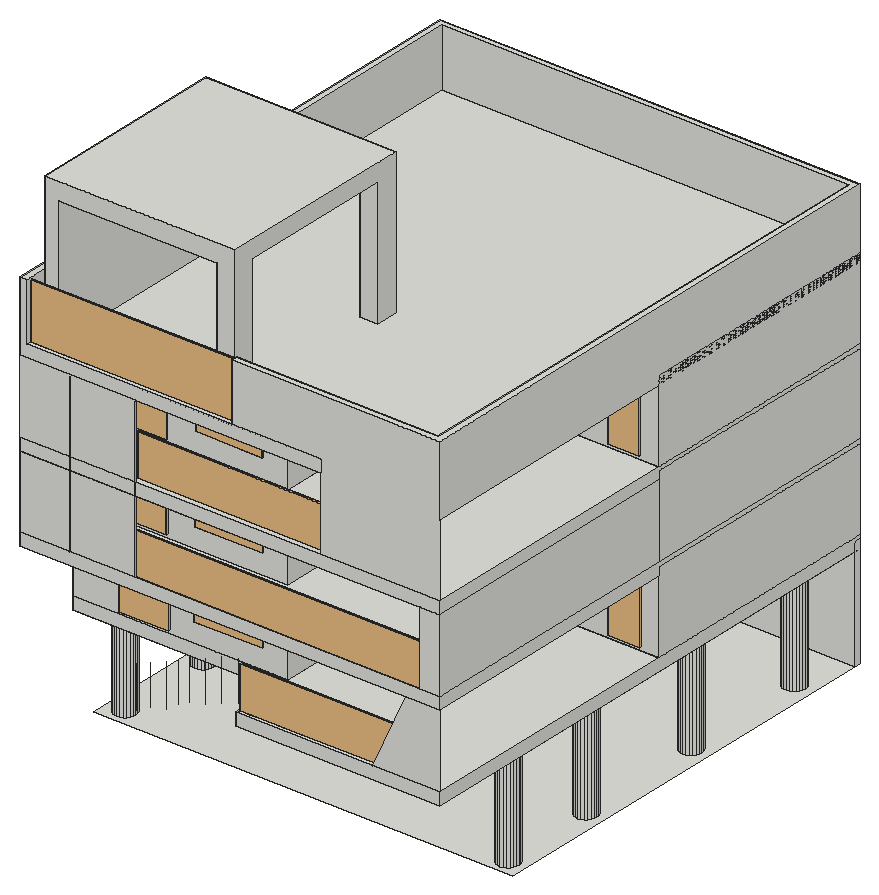
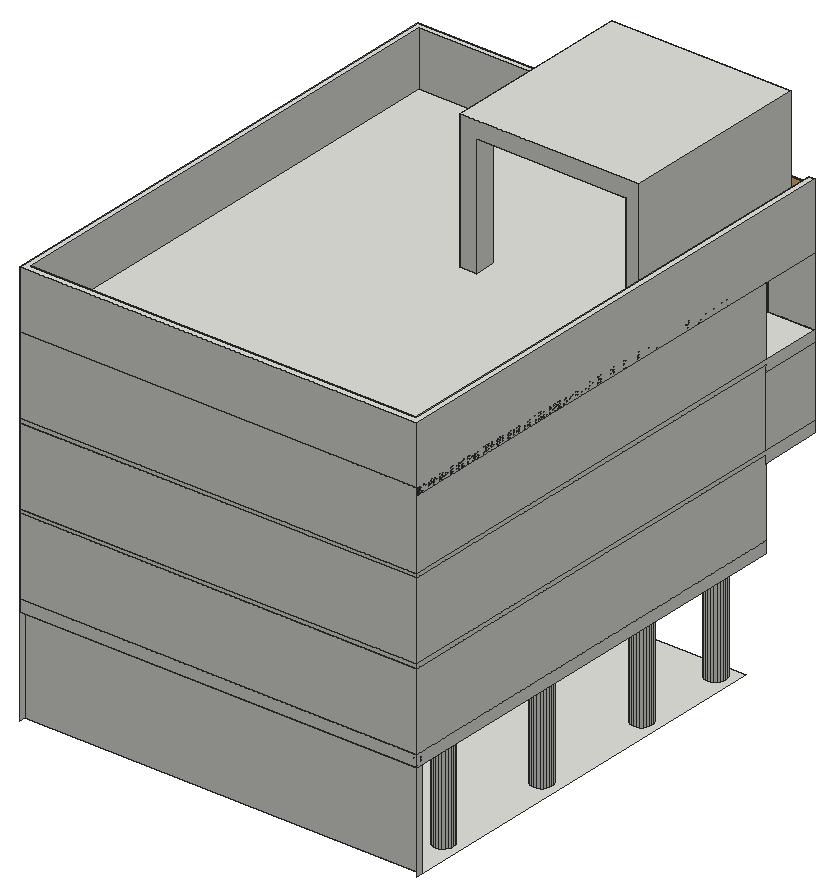
# SketchUp Ruby script. Lengths in millimetres.
U = 1.mm
M = Sketchup.active_model
def pt(a) = Geom::Point3d.new(a.map { |v| v * U })
def face(e, loops, mat)
  f = e.add_face(loops[0].map { |a| pt(a) })
  loops[1..].each { |l| e.add_face(l.map { |a| pt(a) }).erase! }
  f.material = f.back_material = mat if mat
  f
end
# faces: each face lists its corners as indices into pts; further lists are holes
def faces(e, pts, list, mat = nil) = list.each { |f| face(e, (f[0].is_a?(Array) ? f : [f]).map { |l| l.map { |i| pts[i] } }, mat) }
# xy, xz, yz: faces in a plane at the given z, y or x. An outline is a flat list of corners, or four numbers for a rectangle; further outlines are holes
def ring(l) = l.size == 4 ? [[l[0], l[1]], [l[2], l[1]], [l[2], l[3]], [l[0], l[3]]] : l.each_slice(2).to_a
def flat(e, list, mat, &to3) = list.each { |f| face(e, (f[0].is_a?(Array) ? f : [f]).map { |l| ring(l).map { |u, v| to3.(u, v) } }, mat) }
def xy(e, z, list, mat = nil) = flat(e, list, mat) { |x, y| [x, y, z] }
def xz(e, y, list, mat = nil) = flat(e, list, mat) { |x, z| [x, y, z] }
def yz(e, x, list, mat = nil) = flat(e, list, mat) { |y, z| [x, y, z] }
def lines(e, pts, list) = list.each { |a, b| e.add_line(pt(pts[a]), pt(pts[b])) }
# prism: a flat outline (further loops are holes) pulled along v
def prism(e, loops, v, mat = nil)
  f = face(e, loops, mat); d = Geom::Vector3d.new(v.map { |x| x * U })
  f.pushpull(f.normal.samedirection?(d) ? d.length : -d.length)
end
def box(e, o, s, mat = nil) = prism(e, [[o, [o[0] + s[0], o[1], o[2]], [o[0] + s[0], o[1] + s[1], o[2]], [o[0], o[1] + s[1], o[2]]]], [0, 0, s[2]], mat)
def at(x, y, z, deg = 0) = Geom::Transformation.translation(pt([x, y, z])) * Geom::Transformation.rotation(ORIGIN, Z_AXIS, deg.degrees)
def axes(o, x, y, z) = Geom::Transformation.new([*x, 0, *y, 0, *z, 0, *pt(o).to_a, 1])
def part(name) = M.definitions.add(name)
# library, detail: a bought-in or finely detailed component or shape, given as its bounding box
def library(name, o, s) = part(name).tap { |d| box(d.entities, o, s) }
def detail(e, o, s) = box(e.add_group.entities, o, s)
def put(e, d, t, mat = nil) = e.add_instance(d, t).tap { |i| i.material = mat if mat }
def group(e, t, mat = nil) = e.add_group.tap { |g| g.transformation = t; g.material = mat if mat }.entities
root = M.entities
c1 = library("Group\#4",[0,0,0],[1209.1,266,2133.6])
c2 = library("Group\#9",[0,0,0],[2586.8,230.4,1524])
c3 = library("Group\#15",[0,0,0],[2557.7,230.4,1524])
c4 = library("Group\#22",[0,0,0],[1872.8,280.1,2203.6])
c5 = library("Group\#29",[0,0,0],[5758.1,80,1549])
c6 = library("CNC Jali design 2",[0,0,0],[3048,27.5,6081.9])
c7 = library("Group\#6",[0,0,0],[1405.4,266,2133.6])
c8 = library("Group\#11",[0,0,0],[2215.9,230.4,1524])
c9 = library("Group\#17",[0,0,0],[2537.7,230.4,1524])
c10 = library("Group\#20",[0,0,0],[1742.8,280.1,2203.6])
c11 = library("Group\#27",[0,0,0],[10733.1,80,1549])
c12 = library("Group\#7",[0,0,0],[1161.1,266,2133.6])
c13 = library("Group\#13",[0,0,0],[2439.5,230.4,1524])
c14 = library("Group\#19",[0,0,0],[2501.6,230.4,1524])
c15 = library("Group\#21",[0,0,0],[1782.8,280.1,2203.6])
c16 = library("Group\#28",[0,0,0],[7058,80,1549])
c17 = library("Group\#23",[0,0,0],[7774,80,939.4])
xy(root,254,[[[720.2,4710,16417.4,20714.5],[15750.9,18372.1,15647.3,18381.1,15549.5,18416.6,15464.2,18476.2,15397.3,18555.8,15353.3,18650.1,15335.1,18752.5,15344.1,18856.1,15379.6,18953.9,15439.2,19039.1,15518.8,19106.1,15613.1,19150.1,15715.5,19168.3,15819.1,19159.3,15916.9,19123.8,16002.1,19064.2,16069.1,18984.6,16113.1,18890.3,16131.3,18787.9,16122.3,18684.3,16086.8,18586.5,16027.2,18501.2,15947.6,18434.3,15853.3,18390.3],[1429.7,8578.8,1326,8587.8,1228.3,8623.3,1143,8682.9,1076.1,8762.5,1032,8856.8,1013.9,8959.2,1022.9,9062.8,1058.4,9160.6,1117.9,9245.9,1197.6,9312.8,1291.8,9356.8,1394.2,9375,1497.9,9366,1595.6,9330.5,1680.9,9270.9,1747.8,9191.3,1791.9,9097,1810,8994.6,1801,8891,1765.5,8793.2,1705.9,8707.9,1626.3,8641,1532.1,8597],[15768.9,8578.8,15665.2,8587.8,15567.5,8623.3,15482.2,8682.9,15415.3,8762.5,15371.2,8856.8,15353.1,8959.2,15362.1,9062.8,15397.6,9160.6,15457.1,9245.9,15536.8,9312.8,15631,9356.8,15733.4,9375,15837.1,9366,15934.8,9330.5,16020.1,9270.9,16087,9191.3,16131.1,9097,16149.2,8994.6,16140.2,8891,16104.7,8793.2,16045.1,8707.9,15965.5,8641,15871.3,8597],[1429.7,18372.1,1326,18381.1,1228.3,18416.6,1143,18476.2,1076.1,18555.8,1032,18650.1,1013.9,18752.5,1022.9,18856.1,1058.4,18953.9,1117.9,19039.1,1197.6,19106.1,1291.8,19150.1,1394.2,19168.3,1497.9,19159.3,1595.6,19123.8,1680.9,19064.2,1747.8,18984.6,1791.9,18890.3,1810,18787.9,1801,18684.3,1765.5,18586.5,1705.9,18501.2,1626.3,18434.3,1532.1,18390.3],[1429.7,4921.2,1326,4930.2,1228.3,4965.7,1143,5025.3,1076.1,5104.9,1032,5199.2,1013.9,5301.6,1022.9,5405.2,1058.4,5503,1117.9,5588.3,1197.6,5655.2,1291.8,5699.2,1394.2,5717.4,1497.9,5708.4,1595.6,5672.9,1680.9,5613.3,1747.8,5533.7,1791.9,5439.4,1810,5337,1801,5233.4,1765.5,5135.6,1705.9,5050.3,1626.3,4983.4,1532.1,4939.4],[15787,4921.2,15683.4,4930.2,15585.6,4965.7,15500.3,5025.3,15433.4,5104.9,15389.4,5199.2,15371.2,5301.6,15380.2,5405.2,15415.7,5503,15475.3,5588.3,15554.9,5655.2,15649.2,5699.2,15751.6,5717.4,15855.2,5708.4,15953,5672.9,16038.3,5613.3,16105.2,5533.7,16149.2,5439.4,16167.4,5337,16158.4,5233.4,16122.9,5135.6,16063.3,5050.3,15983.7,4983.4,15889.4,4939.4],[15759.9,13504.8,15656.2,13513.8,15558.5,13549.3,15473.2,13608.9,15406.3,13688.5,15362.2,13782.8,15344.1,13885.2,15353.1,13988.8,15388.6,14086.6,15448.2,14171.9,15527.8,14238.8,15622,14282.8,15724.5,14301,15828.1,14292,15925.9,14256.5,16011.1,14196.9,16078.1,14117.3,16122.1,14023,16140.2,13920.6,16131.3,13817,16095.8,13719.2,16036.2,13634,15956.5,13567,15862.3,13523],[1429.7,13504.8,1326,13513.8,1228.3,13549.3,1143,13608.9,1076.1,13688.5,1032,13782.8,1013.9,13885.2,1022.9,13988.8,1058.4,14086.6,1117.9,14171.9,1197.6,14238.8,1291.8,14282.8,1394.2,14301,1497.9,14292,1595.6,14256.5,1680.9,14196.9,1747.8,14117.3,1791.9,14023,1810,13920.6,1801,13817,1765.5,13719.2,1705.9,13634,1626.3,13567,1532.1,13523]]])
xy(root,4419.6,[[1429.7,4921.2,1532.1,4939.4,1626.3,4983.4,1705.9,5050.3,1765.5,5135.6,1801,5233.4,1810,5337,1791.9,5439.4,1747.8,5533.7,1680.9,5613.3,1595.6,5672.9,1497.9,5708.4,1394.2,5717.4,1291.8,5699.2,1197.6,5655.2,1117.9,5588.3,1058.4,5503,1022.9,5405.2,1013.9,5301.6,1032,5199.2,1076.1,5104.9,1143,5025.3,1228.3,4965.7,1326,4930.2],[15787,4921.2,15889.4,4939.4,15983.7,4983.4,16063.3,5050.3,16122.9,5135.6,16158.4,5233.4,16167.4,5337,16149.2,5439.4,16105.2,5533.7,16038.3,5613.3,15953,5672.9,15855.2,5708.4,15751.6,5717.4,15649.2,5699.2,15554.9,5655.2,15475.3,5588.3,15415.7,5503,15380.2,5405.2,15371.2,5301.6,15389.4,5199.2,15433.4,5104.9,15500.3,5025.3,15585.6,4965.7,15683.4,4930.2],[1429.7,8578.8,1532.1,8597,1626.3,8641,1705.9,8707.9,1765.5,8793.2,1801,8891,1810,8994.6,1791.9,9097,1747.8,9191.3,1680.9,9270.9,1595.6,9330.5,1497.9,9366,1394.2,9375,1291.8,9356.8,1197.6,9312.8,1117.9,9245.9,1058.4,9160.6,1022.9,9062.8,1013.9,8959.2,1032,8856.8,1076.1,8762.5,1143,8682.9,1228.3,8623.3,1326,8587.8],[15768.9,8578.8,15871.3,8597,15965.5,8641,16045.1,8707.9,16104.7,8793.2,16140.2,8891,16149.2,8994.6,16131.1,9097,16087,9191.3,16020.1,9270.9,15934.8,9330.5,15837.1,9366,15733.4,9375,15631,9356.8,15536.8,9312.8,15457.1,9245.9,15397.6,9160.6,15362.1,9062.8,15353.1,8959.2,15371.2,8856.8,15415.3,8762.5,15482.2,8682.9,15567.5,8623.3,15665.2,8587.8],[1429.7,13504.8,1532.1,13523,1626.3,13567,1705.9,13634,1765.5,13719.2,1801,13817,1810,13920.6,1791.9,14023,1747.8,14117.3,1680.9,14196.9,1595.6,14256.5,1497.9,14292,1394.2,14301,1291.8,14282.8,1197.6,14238.8,1117.9,14171.9,1058.4,14086.6,1022.9,13988.8,1013.9,13885.2,1032,13782.8,1076.1,13688.5,1143,13608.9,1228.3,13549.3,1326,13513.8],
  [15759.9,13504.8,15862.3,13523,15956.5,13567,16036.2,13634,16095.8,13719.2,16131.3,13817,16140.2,13920.6,16122.1,14023,16078.1,14117.3,16011.1,14196.9,15925.9,14256.5,15828.1,14292,15724.5,14301,15622,14282.8,15527.8,14238.8,15448.2,14171.9,15388.6,14086.6,15353.1,13988.8,15344.1,13885.2,15362.2,13782.8,15406.3,13688.5,15473.2,13608.9,15558.5,13549.3,15656.2,13513.8],[1429.7,18372.1,1532.1,18390.3,1626.3,18434.3,1705.9,18501.2,1765.5,18586.5,1801,18684.3,1810,18787.9,1791.9,18890.3,1747.8,18984.6,1680.9,19064.2,1595.6,19123.8,1497.9,19159.3,1394.2,19168.3,1291.8,19150.1,1197.6,19106.1,1117.9,19039.1,1058.4,18953.9,1022.9,18856.1,1013.9,18752.5,1032,18650.1,1076.1,18555.8,1143,18476.2,1228.3,18416.6,1326,18381.1],[15750.9,18372.1,15853.3,18390.3,15947.6,18434.3,16027.2,18501.2,16086.8,18586.5,16122.3,18684.3,16131.3,18787.9,16113.1,18890.3,16069.1,18984.6,16002.1,19064.2,15916.9,19123.8,15819.1,19159.3,15715.5,19168.3,15613.1,19150.1,15518.8,19106.1,15439.2,19039.1,15379.6,18953.9,15344.1,18856.1,15335.1,18752.5,15353.3,18650.1,15397.3,18555.8,15464.2,18476.2,15549.5,18416.6,15647.3,18381.1],[720.2,20714.5,16417.4,20943.1]])
xy(root,7315.2,[[720.2,1283.5,720.2,3721.9,8797.4,3721.9,8797.4,11570.5,16417.4,11570.5,16417.4,1283.5]])
xy(root,7620,[[720.2,3721.9,720.2,20943.1,16417.4,20943.1,16417.4,11570.5,8797.4,11570.5,8797.4,3721.9]])
xy(root,7772.4,[[720.2,1283.5,16417.4,20943.1]])
xy(root,10515.6,[[720.2,1283.5,720.2,3721.9,8797.4,3721.9,8797.4,11570.5,16417.4,11570.5,16417.4,1283.5]])
xy(root,10820.4,[[720.2,3721.9,720.2,20943.1,16417.4,20943.1,16417.4,11570.5,8797.4,11570.5,8797.4,3721.9]])
xy(root,10972.8,[[720.2,1283.5,16417.4,20943.1]])
xy(root,14173.2,[[948.8,1283.5,8635.5,1512.1],[948.8,1512.1,16188.8,20714.5]])
xy(root,16333.8,[[720.2,1283.5,948.8,1283.5,948.8,20714.5,16188.8,20714.5,16188.8,1512.1,8635.5,1512.1,8635.5,1283.5,16417.4,1283.5,16417.4,20943.1,720.2,20943.1]])
xz(root,1283.5,[[13937.6,4572,16417.4,4572,16417.4,7315.2,15177.5,7315.2],[720.2,7315.2,16417.4,7772.4],[720.2,7772.4,5011.5,10515.6],[15680.9,7772.4,16417.4,10515.6],[720.2,10515.6,16417.4,10972.8],
  [720.2,10972.8,5011.5,13716],[11969.3,10972.8,16417.4,10972.8,16417.4,16333.8,8635.5,16333.8,8635.5,14173.2,11969.3,14173.2],[720.2,13716,11969.3,13716,11969.3,14173.2,948.8,14173.2,948.8,16333.8,720.2,16333.8]])
xz(root,1512.1,[[8635.5,14173.2,16188.8,16333.8]])
xz(root,3721.9,[[720.2,7315.2,8797.4,7620],[720.2,10515.6,8797.4,10820.4]])
xz(root,11570.5,[[8797.4,7315.2,16417.4,7620],[8797.4,10515.6,16417.4,10820.4]])
xz(root,20714.5,[[720.2,254,16417.4,4419.6],[948.8,14173.2,16188.8,16333.8]])
xz(root,20943.1,[[720.2,7620,16417.4,7772.4],[720.2,10820.4,16417.4,10972.8],[720.2,13716,16417.4,16333.8]])
yz(root,720.2,[[20714.5,254,20943.1,4419.6],[1283.5,7315.2,1283.5,7772.4,20943.1,7772.4,20943.1,7620,3721.9,7620,3721.9,7315.2],[1283.5,7772.4,3721.9,10515.6],[1283.5,10515.6,1283.5,10972.8,20943.1,10972.8,20943.1,10820.4,3721.9,10820.4,3721.9,10515.6],[1283.5,13716,20943.1,16333.8]])
yz(root,948.8,[[1283.5,14173.2,20714.5,16333.8]])
yz(root,8635.5,[[1283.5,14173.2,1512.1,16333.8]])
yz(root,8797.4,[[3721.9,7315.2,11570.5,7620],[3721.9,10515.6,11570.5,10820.4]])
yz(root,16188.8,[[1512.1,14173.2,20714.5,16333.8]])
yz(root,16417.4,[[20714.5,254,20943.1,4419.6],[1283.5,7315.2,11570.5,7315.2,11570.5,7620,20943.1,7620,20943.1,7772.4,1283.5,7772.4],[1283.5,7772.4,11570.5,10515.6],[1283.5,10515.6,11570.5,10515.6,11570.5,10820.4,20943.1,10820.4,20943.1,10972.8,1283.5,10972.8],[1283.5,13716,20943.1,16333.8]])
p = [[1429.7,4921.2,4419.6],[1326,4930.2,4419.6],[1326,4930.2,254],[1429.7,4921.2,254],[1532.1,4939.4,4419.6],[1532.1,4939.4,254],
  [15787,4921.2,4419.6],[15683.4,4930.2,4419.6],[15683.4,4930.2,254],[15787,4921.2,254],[15889.4,4939.4,4419.6],[15889.4,4939.4,254],
  [1228.3,4965.7,4419.6],[1228.3,4965.7,254],[15585.6,4965.7,4419.6],[15585.6,4965.7,254],[1626.3,4983.4,4419.6],[1626.3,4983.4,254],
  [15983.7,4983.4,4419.6],[15983.7,4983.4,254],[1143,5025.3,4419.6],[1143,5025.3,254],[15500.3,5025.3,4419.6],[15500.3,5025.3,254],
  [1705.9,5050.3,4419.6],[1705.9,5050.3,254],[16063.3,5050.3,4419.6],[16063.3,5050.3,254],[1076.1,5104.9,4419.6],[1076.1,5104.9,254],
  [15433.4,5104.9,4419.6],[15433.4,5104.9,254],[1765.5,5135.6,4419.6],[1765.5,5135.6,254],[16122.9,5135.6,4419.6],[16122.9,5135.6,254],
  [1032,5199.2,4419.6],[1032,5199.2,254],[15389.4,5199.2,4419.6],[15389.4,5199.2,254],[1801,5233.4,4419.6],[1801,5233.4,254],
  [16158.4,5233.4,4419.6],[16158.4,5233.4,254],[1013.9,5301.6,4419.6],[1013.9,5301.6,254],[15371.2,5301.6,4419.6],[15371.2,5301.6,254],
  [1810,5337,4419.6],[1810,5337,254],[16167.4,5337,4419.6],[16167.4,5337,254],[1022.9,5405.2,4419.6],[1022.9,5405.2,254],
  [15380.2,5405.2,4419.6],[15380.2,5405.2,254],[1791.9,5439.4,4419.6],[1791.9,5439.4,254],[16149.2,5439.4,4419.6],[16149.2,5439.4,254],
  [1058.4,5503,4419.6],[1058.4,5503,254],[15415.7,5503,4419.6],[15415.7,5503,254],[1747.8,5533.7,4419.6],[1747.8,5533.7,254],
  [16105.2,5533.7,4419.6],[16105.2,5533.7,254],[1117.9,5588.3,4419.6],[1117.9,5588.3,254],[15475.3,5588.3,4419.6],[15475.3,5588.3,254],
  [1680.9,5613.3,4419.6],[1680.9,5613.3,254],[16038.3,5613.3,4419.6],[16038.3,5613.3,254],[1197.6,5655.2,4419.6],[1197.6,5655.2,254],
  [15554.9,5655.2,4419.6],[15554.9,5655.2,254],[1595.6,5672.9,4419.6],[1595.6,5672.9,254],[15953,5672.9,4419.6],[15953,5672.9,254],
  [1291.8,5699.2,4419.6],[1291.8,5699.2,254],[15649.2,5699.2,4419.6],[15649.2,5699.2,254],[1497.9,5708.4,4419.6],[1497.9,5708.4,254],
  [15855.2,5708.4,4419.6],[15855.2,5708.4,254],[1394.2,5717.4,4419.6],[1394.2,5717.4,254],[15751.6,5717.4,4419.6],[15751.6,5717.4,254],
  [1429.7,8578.8,4419.6],[1326,8587.8,4419.6],[1326,8587.8,254],[1429.7,8578.8,254],[1532.1,8597,4419.6],[1532.1,8597,254],
  [15768.9,8578.8,4419.6],[15665.2,8587.8,4419.6],[15665.2,8587.8,254],[15768.9,8578.8,254],[15871.3,8597,4419.6],[15871.3,8597,254],
  [1228.3,8623.3,4419.6],[1228.3,8623.3,254],[15567.5,8623.3,4419.6],[15567.5,8623.3,254],[1626.3,8641,4419.6],[1626.3,8641,254],
  [15965.5,8641,4419.6],[15965.5,8641,254],[1143,8682.9,4419.6],[1143,8682.9,254],[15482.2,8682.9,4419.6],[15482.2,8682.9,254],
  [1705.9,8707.9,4419.6],[1705.9,8707.9,254],[16045.1,8707.9,4419.6],[16045.1,8707.9,254],[1076.1,8762.5,4419.6],[1076.1,8762.5,254],
  [15415.3,8762.5,4419.6],[15415.3,8762.5,254],[1765.5,8793.2,4419.6],[1765.5,8793.2,254],[16104.7,8793.2,4419.6],[16104.7,8793.2,254],
  [1032,8856.8,4419.6],[1032,8856.8,254],[15371.2,8856.8,4419.6],[15371.2,8856.8,254],[1801,8891,4419.6],[1801,8891,254],
  [16140.2,8891,4419.6],[16140.2,8891,254],[1013.9,8959.2,4419.6],[1013.9,8959.2,254],[15353.1,8959.2,4419.6],[15353.1,8959.2,254],
  [1810,8994.6,4419.6],[1810,8994.6,254],[16149.2,8994.6,4419.6],[16149.2,8994.6,254],[1022.9,9062.8,4419.6],[1022.9,9062.8,254],
  [15362.1,9062.8,4419.6],[15362.1,9062.8,254],[1791.9,9097,4419.6],[1791.9,9097,254],[16131.1,9097,4419.6],[16131.1,9097,254],
  [1058.4,9160.6,4419.6],[1058.4,9160.6,254],[15397.6,9160.6,4419.6],[15397.6,9160.6,254],[1747.8,9191.3,4419.6],[1747.8,9191.3,254],
  [16087,9191.3,4419.6],[16087,9191.3,254],[1117.9,9245.9,4419.6],[1117.9,9245.9,254],[15457.1,9245.9,4419.6],[15457.1,9245.9,254],
  [1680.9,9270.9,4419.6],[1680.9,9270.9,254],[16020.1,9270.9,4419.6],[16020.1,9270.9,254],[1197.6,9312.8,4419.6],[1197.6,9312.8,254],
  [15536.8,9312.8,4419.6],[15536.8,9312.8,254],[1595.6,9330.5,4419.6],[1595.6,9330.5,254],[15934.8,9330.5,4419.6],[15934.8,9330.5,254],
  [1291.8,9356.8,4419.6],[1291.8,9356.8,254],[15631,9356.8,4419.6],[15631,9356.8,254],[1497.9,9366,4419.6],[1497.9,9366,254],
  [15837.1,9366,4419.6],[15837.1,9366,254],[1394.2,9375,4419.6],[1394.2,9375,254],[15733.4,9375,4419.6],[15733.4,9375,254],
  [1429.7,13504.8,4419.6],[1326,13513.8,4419.6],[1326,13513.8,254],[1429.7,13504.8,254],[1532.1,13523,4419.6],[1532.1,13523,254],
  [15759.9,13504.8,4419.6],[15656.2,13513.8,4419.6],[15656.2,13513.8,254],[15759.9,13504.8,254],[15862.3,13523,4419.6],[15862.3,13523,254],
  [1228.3,13549.3,4419.6],[1228.3,13549.3,254],[15558.5,13549.3,4419.6],[15558.5,13549.3,254],[1626.3,13567,4419.6],[1626.3,13567,254],
  [15956.5,13567,4419.6],[15956.5,13567,254],[1143,13608.9,4419.6],[1143,13608.9,254],[15473.2,13608.9,4419.6],[15473.2,13608.9,254],
  [1705.9,13634,4419.6],[1705.9,13634,254],[16036.2,13634,4419.6],[16036.2,13634,254],[1076.1,13688.5,4419.6],[1076.1,13688.5,254],
  [15406.3,13688.5,4419.6],[15406.3,13688.5,254],[1765.5,13719.2,4419.6],[1765.5,13719.2,254],[16095.8,13719.2,4419.6],[16095.8,13719.2,254],
  [1032,13782.8,4419.6],[1032,13782.8,254],[15362.2,13782.8,4419.6],[15362.2,13782.8,254],[1801,13817,4419.6],[1801,13817,254],
  [16131.3,13817,4419.6],[16131.3,13817,254],[1013.9,13885.2,4419.6],[1013.9,13885.2,254],[15344.1,13885.2,4419.6],[15344.1,13885.2,254],
  [1810,13920.6,4419.6],[1810,13920.6,254],[16140.2,13920.6,4419.6],[16140.2,13920.6,254],[1022.9,13988.8,4419.6],[1022.9,13988.8,254],
  [15353.1,13988.8,4419.6],[15353.1,13988.8,254],[1791.9,14023,4419.6],[1791.9,14023,254],[16122.1,14023,4419.6],[16122.1,14023,254],
  [1058.4,14086.6,4419.6],[1058.4,14086.6,254],[15388.6,14086.6,4419.6],[15388.6,14086.6,254],[1747.8,14117.3,4419.6],[1747.8,14117.3,254],
  [16078.1,14117.3,4419.6],[16078.1,14117.3,254],[1117.9,14171.9,4419.6],[1117.9,14171.9,254],[15448.2,14171.9,4419.6],[15448.2,14171.9,254],
  [1680.9,14196.9,4419.6],[1680.9,14196.9,254],[16011.1,14196.9,4419.6],[16011.1,14196.9,254],[1197.6,14238.8,4419.6],[1197.6,14238.8,254],
  [15527.8,14238.8,4419.6],[15527.8,14238.8,254],[1595.6,14256.5,4419.6],[1595.6,14256.5,254],[15925.9,14256.5,4419.6],[15925.9,14256.5,254],
  [1291.8,14282.8,4419.6],[1291.8,14282.8,254],[15622,14282.8,4419.6],[15622,14282.8,254],[1497.9,14292,4419.6],[1497.9,14292,254],
  [15828.1,14292,4419.6],[15828.1,14292,254],[1394.2,14301,4419.6],[1394.2,14301,254],[15724.5,14301,4419.6],[15724.5,14301,254],
  [1429.7,18372.1,4419.6],[1326,18381.1,4419.6],[1326,18381.1,254],[1429.7,18372.1,254],[1532.1,18390.3,4419.6],[1532.1,18390.3,254],
  [15750.9,18372.1,4419.6],[15647.3,18381.1,4419.6],[15647.3,18381.1,254],[15750.9,18372.1,254],[15853.3,18390.3,4419.6],[15853.3,18390.3,254],
  [1228.3,18416.6,4419.6],[1228.3,18416.6,254],[15549.5,18416.6,4419.6],[15549.5,18416.6,254],[1626.3,18434.3,4419.6],[1626.3,18434.3,254],
  [15947.6,18434.3,4419.6],[15947.6,18434.3,254],[1143,18476.2,4419.6],[1143,18476.2,254],[15464.2,18476.2,4419.6],[15464.2,18476.2,254],
  [1705.9,18501.2,4419.6],[1705.9,18501.2,254],[16027.2,18501.2,4419.6],[16027.2,18501.2,254],[1076.1,18555.8,4419.6],[1076.1,18555.8,254],
  [15397.3,18555.8,4419.6],[15397.3,18555.8,254],[1765.5,18586.5,4419.6],[1765.5,18586.5,254],[16086.8,18586.5,4419.6],[16086.8,18586.5,254],
  [1032,18650.1,4419.6],[1032,18650.1,254],[15353.3,18650.1,4419.6],[15353.3,18650.1,254],[1801,18684.3,4419.6],[1801,18684.3,254],
  [16122.3,18684.3,4419.6],[16122.3,18684.3,254],[1013.9,18752.5,4419.6],[1013.9,18752.5,254],[15335.1,18752.5,4419.6],[15335.1,18752.5,254],
  [1810,18787.9,4419.6],[1810,18787.9,254],[16131.3,18787.9,4419.6],[16131.3,18787.9,254],[1022.9,18856.1,4419.6],[1022.9,18856.1,254],
  [15344.1,18856.1,4419.6],[15344.1,18856.1,254],[1791.9,18890.3,4419.6],[1791.9,18890.3,254],[16113.1,18890.3,4419.6],[16113.1,18890.3,254],
  [1058.4,18953.9,4419.6],[1058.4,18953.9,254],[15379.6,18953.9,4419.6],[15379.6,18953.9,254],[1747.8,18984.6,4419.6],[1747.8,18984.6,254],
  [16069.1,18984.6,4419.6],[16069.1,18984.6,254],[1117.9,19039.1,4419.6],[1117.9,19039.1,254],[15439.2,19039.1,4419.6],[15439.2,19039.1,254],
  [1680.9,19064.2,4419.6],[1680.9,19064.2,254],[16002.1,19064.2,4419.6],[16002.1,19064.2,254],[1197.6,19106.1,4419.6],[1197.6,19106.1,254],
  [15518.8,19106.1,4419.6],[15518.8,19106.1,254],[1595.6,19123.8,4419.6],[1595.6,19123.8,254],[15916.9,19123.8,4419.6],[15916.9,19123.8,254],
  [1291.8,19150.1,4419.6],[1291.8,19150.1,254],[15613.1,19150.1,4419.6],[15613.1,19150.1,254],[1497.9,19159.3,4419.6],[1497.9,19159.3,254],
  [15819.1,19159.3,4419.6],[15819.1,19159.3,254],[1394.2,19168.3,4419.6],[1394.2,19168.3,254],[15715.5,19168.3,4419.6],[15715.5,19168.3,254],
  [8797.4,3721.9,13716],[720.2,3721.9,13716],[6265.9,1734,5229.9],[6265.9,1734,3758.3],[5841.1,1734,5049.3],[5841.1,1734,3446.3],
  [5247.8,1734,4797.1],[5247.8,1734,3295.5],[6703.4,1734,5415.8],[6703.4,1734,3963.3],[7882.6,1734,5917.1],[7882.6,1734,4346.9],
  [8532.6,1734,6080.9],[8532.6,1734,4572],[7296.2,1734,5667.9],[7296.2,1734,4121.7],[4718.2,1734,4572],[4718.2,1734,2996],
  [4213.3,1734,4357.3],[4213.3,1734,2770.9],[3796.2,1734,4180.1],[3796.2,1734,2545.8],[13925.3,1488.1,4572],[8875.5,1488.1,4572]]
faces(root,p,[[0,1,2,3],[4,0,3,5],[6,7,8,9],[10,6,9,11],[1,12,13,2],[7,14,15,8],[16,4,5,17],[18,10,11,19],
  [12,20,21,13],[14,22,23,15],[24,16,17,25],[26,18,19,27],[20,28,29,21],[22,30,31,23],[32,24,25,33],[34,26,27,35],
  [28,36,37,29],[30,38,39,31],[40,32,33,41],[42,34,35,43],[36,44,45,37],[38,46,47,39],[48,40,41,49],[50,42,43,51],
  [44,52,53,45],[46,54,55,47],[56,48,49,57],[58,50,51,59],[52,60,61,53],[54,62,63,55],[64,56,57,65],[66,58,59,67],
  [60,68,69,61],[62,70,71,63],[72,64,65,73],[74,66,67,75],[68,76,77,69],[70,78,79,71],[80,72,73,81],[82,74,75,83],
  [76,84,85,77],[78,86,87,79],[88,80,81,89],[90,82,83,91],[84,92,93,85],[86,94,95,87],[92,88,89,93],[94,90,91,95],
  [96,97,98,99],[100,96,99,101],[102,103,104,105],[106,102,105,107],[97,108,109,98],[103,110,111,104],[112,100,101,113],[114,106,107,115],
  [108,116,117,109],[110,118,119,111],[120,112,113,121],[122,114,115,123],[116,124,125,117],[118,126,127,119],[128,120,121,129],[130,122,123,131],
  [124,132,133,125],[126,134,135,127],[136,128,129,137],[138,130,131,139],[132,140,141,133],[134,142,143,135],[144,136,137,145],[146,138,139,147],
  [140,148,149,141],[142,150,151,143],[152,144,145,153],[154,146,147,155],[148,156,157,149],[150,158,159,151],[160,152,153,161],[162,154,155,163],
  [156,164,165,157],[158,166,167,159],[168,160,161,169],[170,162,163,171],[164,172,173,165],[166,174,175,167],[176,168,169,177],[178,170,171,179],
  [172,180,181,173],[174,182,183,175],[184,176,177,185],[186,178,179,187],[180,188,189,181],[182,190,191,183],[188,184,185,189],[190,186,187,191],
  [192,193,194,195],[196,192,195,197],[198,199,200,201],[202,198,201,203],[193,204,205,194],[199,206,207,200],[208,196,197,209],[210,202,203,211],
  [204,212,213,205],[206,214,215,207],[216,208,209,217],[218,210,211,219],[212,220,221,213],[214,222,223,215],[224,216,217,225],[226,218,219,227],
  [220,228,229,221],[222,230,231,223],[232,224,225,233],[234,226,227,235],[228,236,237,229],[230,238,239,231],[240,232,233,241],[242,234,235,243],
  [236,244,245,237],[238,246,247,239],[248,240,241,249],[250,242,243,251],[244,252,253,245],[246,254,255,247],[256,248,249,257],[258,250,251,259],
  [252,260,261,253],[254,262,263,255],[264,256,257,265],[266,258,259,267],[260,268,269,261],[262,270,271,263],[272,264,265,273],[274,266,267,275],
  [268,276,277,269],[270,278,279,271],[280,272,273,281],[282,274,275,283],[276,284,285,277],[278,286,287,279],[284,280,281,285],[286,282,283,287],
  [288,289,290,291],[292,288,291,293],[294,295,296,297],[298,294,297,299],[289,300,301,290],[295,302,303,296],[304,292,293,305],[306,298,299,307],
  [300,308,309,301],[302,310,311,303],[312,304,305,313],[314,306,307,315],[308,316,317,309],[310,318,319,311],[320,312,313,321],[322,314,315,323],
  [316,324,325,317],[318,326,327,319],[328,320,321,329],[330,322,323,331],[324,332,333,325],[326,334,335,327],[336,328,329,337],[338,330,331,339],
  [332,340,341,333],[334,342,343,335],[344,336,337,345],[346,338,339,347],[340,348,349,341],[342,350,351,343],[352,344,345,353],[354,346,347,355],
  [348,356,357,349],[350,358,359,351],[360,352,353,361],[362,354,355,363],[356,364,365,357],[358,366,367,359],[368,360,361,369],[370,362,363,371],
  [364,372,373,365],[366,374,375,367],[376,368,369,377],[378,370,371,379],[372,380,381,373],[374,382,383,375],[380,376,377,381],[382,378,379,383]])
lines(root,p,[[384,385],[386,387],[388,389],[390,391],[392,393],[394,395],[396,397],[398,399],[400,401],[402,403],[404,405],[406,407]])
g1 = group(root,at(720.2,3721.9,4419.6))
xy(g1,-304.8,[[8077.2,-2438.4,8077.2,0,0,0,0,17221.2,15697.2,17221.2,15697.2,-2438.4]])
xy(g1,152.4,[[8077.2,-2438.4,15697.2,7848.6],[0,0,8077.2,0,8077.2,7848.6,15697.2,7848.6,15697.2,17221.2,0,17221.2]])
xz(g1,-2438.4,[[8077.2,-304.8,15697.2,152.4]])
xz(g1,0,[[0,-304.8,8077.2,152.4]])
xz(g1,17221.2,[[0,-304.8,15697.2,152.4]])
yz(g1,0,[[0,-304.8,17221.2,152.4]])
yz(g1,8077.2,[[-2438.4,-304.8,0,152.4]])
yz(g1,15697.2,[[-2438.4,-304.8,17221.2,152.4]])
g2 = group(root,at(720.2,3721.9,4572))
xy(g2,0,[[0,0,0,17221.2,15697.2,17221.2,15697.2,7848.6,8077.2,7848.6,8077.2,228.6,7848.6,228.6,7848.6,8077.2,15468.6,8077.2,15468.6,16992.6,228.6,16992.6,228.6,228.6,8077.2,228.6,8077.2,0],[228.6,228.6,7848.6,228.6,7848.6,8077.2,15468.6,8077.2,15468.6,16992.6,228.6,16992.6]])
xy(g2,101.6,[[1842.7,0,3575.5,228.6],[13795.2,7848.6,15004.3,8077.2]])
xy(g2,736.6,[[4559.4,0,7117.1,228.6],[10531.6,7848.6,13118.3,8077.2]])
xy(g2,2235.2,[[1842.7,0,3575.5,228.6],[13795.2,7848.6,15004.3,8077.2]])
xy(g2,2260.6,[[4559.4,0,7117.1,228.6],[10531.6,7848.6,13118.3,8077.2]])
xy(g2,3048,[[[0,0,8077.2,0,8077.2,7848.6,15697.2,7848.6,15697.2,17221.2,0,17221.2],[228.6,228.6,228.6,16992.6,15468.6,16992.6,15468.6,8077.2,7848.6,8077.2,7848.6,228.6]]])
xz(g2,0,[[[0,0,8077.2,3048],[4559.4,736.6,7117.1,2260.6],[1842.7,101.6,3575.5,2235.2]]])
xz(g2,228.6,[[[228.6,0,7848.6,3048],[4559.4,736.6,7117.1,2260.6],[1842.7,101.6,3575.5,2235.2]]])
xz(g2,7848.6,[[[8077.2,0,15697.2,3048],[10531.6,736.6,13118.3,2260.6],[13795.2,101.6,15004.3,2235.2]]])
xz(g2,8077.2,[[[7848.6,0,15468.6,3048],[10531.6,736.6,13118.3,2260.6],[13795.2,101.6,15004.3,2235.2]]])
xz(g2,16992.6,[[228.6,0,15468.6,3048]])
xz(g2,17221.2,[[0,0,15697.2,3048]])
yz(g2,0,[[0,0,17221.2,3048]])
yz(g2,228.6,[[228.6,0,16992.6,3048]])
yz(g2,1842.7,[[0,101.6,228.6,2235.2]])
yz(g2,3575.5,[[0,101.6,228.6,2235.2]])
yz(g2,4559.4,[[0,736.6,228.6,2260.6]])
yz(g2,7117.1,[[0,736.6,228.6,2260.6]])
yz(g2,7848.6,[[228.6,0,8077.2,3048]])
yz(g2,8077.2,[[0,0,7848.6,3048]])
yz(g2,10531.6,[[7848.6,736.6,8077.2,2260.6]])
yz(g2,13118.3,[[7848.6,736.6,8077.2,2260.6]])
yz(g2,13795.2,[[7848.6,101.6,8077.2,2235.2]])
yz(g2,15004.3,[[7848.6,101.6,8077.2,2235.2]])
yz(g2,15468.6,[[8077.2,0,16992.6,3048]])
yz(g2,15697.2,[[7848.6,0,17221.2,3048]])
put(g2,c1,at(13795.2,7811.2,101.6))
put(g2,c2,at(13118.3,8077.2,736.6,180))
put(g2,c3,at(7117.1,228.6,736.6,180))
put(g2,c4,at(1772.7,-30,101.6))
put(root,c5,axes([8825.5,1448.1,4572],[1.01,0,0],[0,1,0],[0,0,1]))
put(root,c6,axes([2562.6,1283.5,7772.4],[0.80344,0,0],[0,0.8,0],[0,0,0.968]))
g3 = group(root,at(720.2,3721.9,7772.4))
xy(g3,0,[[0,0,0,17221.2,15697.2,17221.2,15697.2,7848.6,8077.2,7848.6,8077.2,228.6,7848.6,228.6,7848.6,8077.2,15468.6,8077.2,15468.6,16992.6,228.6,16992.6,228.6,228.6,8077.2,228.6,8077.2,0],[228.6,228.6,7848.6,228.6,7848.6,8077.2,15468.6,8077.2,15468.6,16992.6,228.6,16992.6]])
xy(g3,101.6,[[1902.7,0,3505.5,228.6],[10248.5,7848.6,11653.9,8077.2]])
xy(g3,736.6,[[4578.4,0,7116.1,228.6],[12365.4,7848.6,14581.4,8077.2]])
xy(g3,2235.2,[[1902.7,0,3505.5,228.6],[10248.5,7848.6,11653.9,8077.2]])
xy(g3,2260.6,[[4578.4,0,7116.1,228.6],[12365.4,7848.6,14581.4,8077.2]])
xy(g3,3048,[[[0,0,8077.2,0,8077.2,7848.6,15697.2,7848.6,15697.2,17221.2,0,17221.2],[228.6,228.6,228.6,16992.6,15468.6,16992.6,15468.6,8077.2,7848.6,8077.2,7848.6,228.6]]])
xz(g3,0,[[[0,0,8077.2,3048],[4578.4,736.6,7116.1,2260.6],[1902.7,101.6,3505.5,2235.2]]])
xz(g3,228.6,[[[228.6,0,7848.6,3048],[4578.4,736.6,7116.1,2260.6],[1902.7,101.6,3505.5,2235.2]]])
xz(g3,7848.6,[[[8077.2,0,15697.2,3048],[12365.4,736.6,14581.4,2260.6],[10248.5,101.6,11653.9,2235.2]]])
xz(g3,8077.2,[[[7848.6,0,15468.6,3048],[8966.2,101.6,11653.9,2235.2],[12365.4,736.6,14581.4,2260.6]]])
xz(g3,16992.6,[[228.6,0,15468.6,3048]])
xz(g3,17221.2,[[0,0,15697.2,3048]])
yz(g3,0,[[0,0,17221.2,3048]])
yz(g3,228.6,[[228.6,0,16992.6,3048]])
yz(g3,1902.7,[[0,101.6,228.6,2235.2]])
yz(g3,3505.5,[[0,101.6,228.6,2235.2]])
yz(g3,4578.4,[[0,736.6,228.6,2260.6]])
yz(g3,7116.1,[[0,736.6,228.6,2260.6]])
yz(g3,7848.6,[[228.6,0,8077.2,3048]])
yz(g3,8077.2,[[0,0,7848.6,3048]])
yz(g3,10248.5,[[7848.6,101.6,8077.2,2235.2]])
yz(g3,11653.9,[[7848.6,101.6,8077.2,2235.2]])
yz(g3,12365.4,[[7848.6,736.6,8077.2,2260.6]])
yz(g3,14581.4,[[7848.6,736.6,8077.2,2260.6]])
yz(g3,15468.6,[[8077.2,0,16992.6,3048]])
yz(g3,15697.2,[[7848.6,0,17221.2,3048]])
p = [[8966.2,7848.6,101.6],[8966.2,8077.2,101.6],[8966.2,7848.6,2235.2],[8966.2,8077.2,2235.2]]
lines(g3,p,[[0,1],[2,3]])
put(g3,c7,at(10248.5,7811.2,101.6))
put(g3,c8,at(12365.4,7848.6,736.6))
put(g3,c9,at(7116.1,228.6,736.6,180))
put(g3,c10,at(1832.7,-30,101.6))
put(root,c11,at(4960.6,1323.2,7772.4))
g4 = group(root,at(720.2,3721.9,10972.8))
xy(g4,0,[[0,0,0,17221.2,15697.2,17221.2,15697.2,7848.6,8077.2,7848.6,8077.2,228.6,7848.6,228.6,7848.6,8077.2,15468.6,8077.2,15468.6,16992.6,228.6,16992.6,228.6,228.6,8077.2,228.6,8077.2,0],[228.6,228.6,7848.6,228.6,7848.6,8077.2,15468.6,8077.2,15468.6,16992.6,228.6,16992.6]])
xy(g4,101.6,[[1842.7,0,3485.5,228.6],[13795.2,7848.6,14956.3,8077.2]])
xy(g4,736.6,[[4613.5,0,7115.1,228.6],[10594.4,7848.6,13033.9,8077.2]])
xy(g4,2235.2,[[1842.7,0,3485.5,228.6],[13795.2,7848.6,14956.3,8077.2]])
xy(g4,2260.6,[[4613.5,0,7115.1,228.6],[10594.4,7848.6,13033.9,8077.2]])
xy(g4,3048,[[[0,0,8077.2,0,8077.2,7848.6,15697.2,7848.6,15697.2,17221.2,0,17221.2],[228.6,228.6,228.6,16992.6,15468.6,16992.6,15468.6,8077.2,7848.6,8077.2,7848.6,228.6]]])
xz(g4,0,[[[0,0,8077.2,3048],[4613.5,736.6,7115.1,2260.6],[1842.7,101.6,3485.5,2235.2]]])
xz(g4,228.6,[[[228.6,0,7848.6,3048],[4613.5,736.6,7115.1,2260.6],[1842.7,101.6,3485.5,2235.2]]])
xz(g4,7848.6,[[[8077.2,0,15697.2,3048],[10594.4,736.6,13033.9,2260.6],[13795.2,101.6,14956.3,2235.2]]])
xz(g4,8077.2,[[[7848.6,0,15468.6,3048],[10594.4,736.6,13033.9,2260.6],[13795.2,101.6,14956.3,2235.2]]])
xz(g4,16992.6,[[228.6,0,15468.6,3048]])
xz(g4,17221.2,[[0,0,15697.2,3048]])
yz(g4,0,[[0,0,17221.2,3048]])
yz(g4,228.6,[[228.6,0,16992.6,3048]])
yz(g4,1842.7,[[0,101.6,228.6,2235.2]])
yz(g4,3485.5,[[0,101.6,228.6,2235.2]])
yz(g4,4613.5,[[0,736.6,228.6,2260.6]])
yz(g4,7115.1,[[0,736.6,228.6,2260.6]])
yz(g4,7848.6,[[228.6,0,8077.2,3048]])
yz(g4,8077.2,[[0,0,7848.6,3048]])
yz(g4,10594.4,[[7848.6,736.6,8077.2,2260.6]])
yz(g4,13033.9,[[7848.6,736.6,8077.2,2260.6]])
yz(g4,13795.2,[[7848.6,101.6,8077.2,2235.2]])
yz(g4,14956.3,[[7848.6,101.6,8077.2,2235.2]])
yz(g4,15468.6,[[8077.2,0,16992.6,3048]])
yz(g4,15697.2,[[7848.6,0,17221.2,3048]])
put(g4,c12,at(13795.2,7811.2,101.6))
put(g4,c13,at(13033.9,8077.2,736.6,180))
put(g4,c14,at(7115.1,228.6,736.6,180))
put(g4,c15,at(1772.7,-30,101.6))
put(root,c16,at(4930.4,1513.7,10972.8))
g5 = group(root,at(1126.4,1943.7,14173.2))
xy(g5,0,[[0,0,515.9,7513.6],[6415.1,6697.7,7100.9,7513.6]])
xy(g5,134.2,[[6415.1,0,7100.9,816]])
xy(g5,4751,[[515.9,0,515.9,7513.6,6415.1,7513.6,6415.1,6697.7,7100.9,6697.7,7100.9,816,6415.1,816,6415.1,0]])
xy(g5,5422.9,[[0,0,7100.9,7513.6]])
xz(g5,0,[[0,0,515.9,0,515.9,4751,6415.1,4751,6415.1,134.2,7100.9,134.2,7100.9,5422.9,0,5422.9]])
xz(g5,816,[[6415.1,134.2,7100.9,4751]])
xz(g5,6697.7,[[6415.1,0,7100.9,4751]])
xz(g5,7513.6,[[0,0,0,5422.9,7100.9,5422.9,7100.9,0,6415.1,0,6415.1,4751,515.9,4751,515.9,0]])
yz(g5,0,[[0,0,7513.6,5422.9]])
yz(g5,515.9,[[0,0,7513.6,4751]])
yz(g5,6415.1,[[6697.7,0,7513.6,4751],[0,134.2,816,4751]])
yz(g5,7100.9,[[6697.7,0,7513.6,0,7513.6,5422.9,0,5422.9,0,134.2,816,134.2,816,4751,6697.7,4751]])
put(root,c17,axes([948.8,1472.1,14173.2],[0.98877,0,0],[0,1,0],[0,0,2.20911]))
